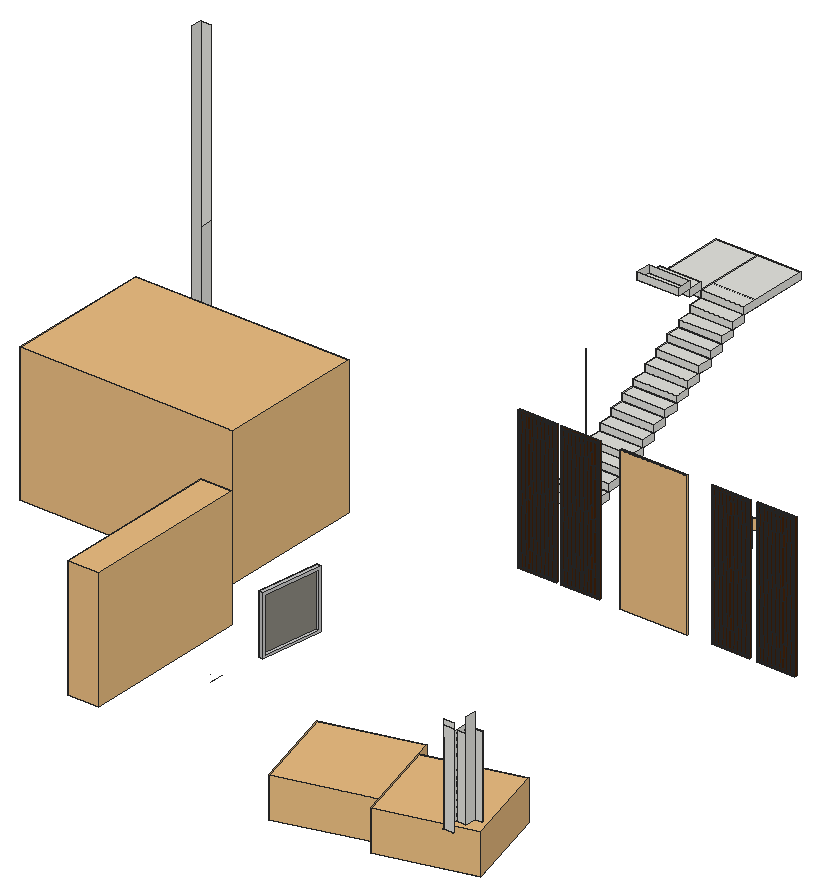
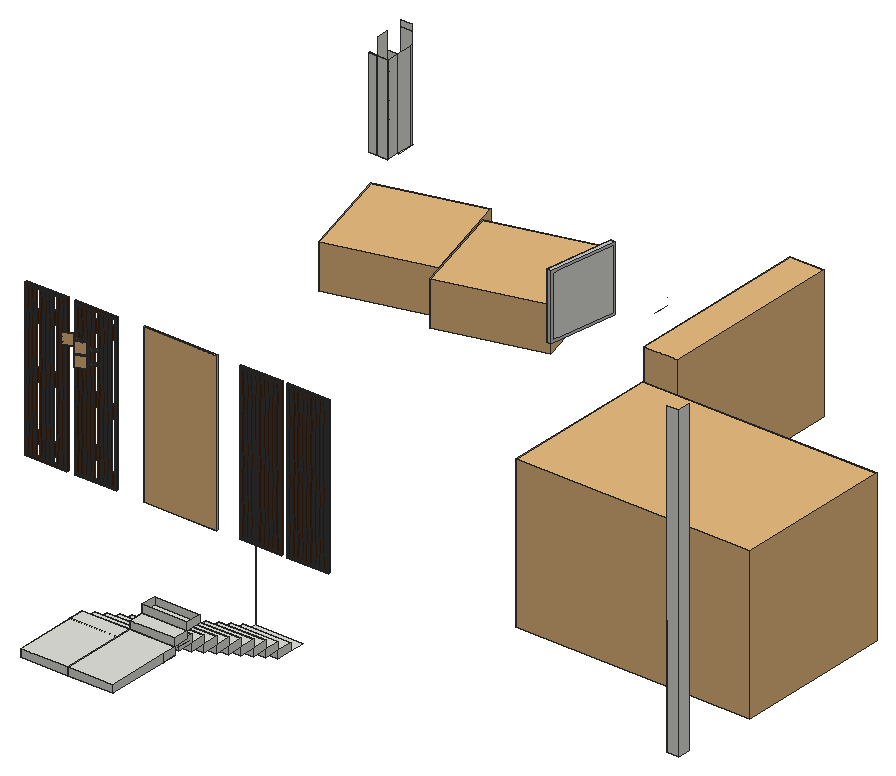
# SketchUp Ruby script. Lengths in inches.
U = 1.inch
M = Sketchup.active_model
def pt(a) = Geom::Point3d.new(a.map { |v| v * U })
def face(e, loops, mat)
  f = e.add_face(loops[0].map { |a| pt(a) })
  loops[1..].each { |l| e.add_face(l.map { |a| pt(a) }).erase! }
  f.material = f.back_material = mat if mat
  f
end
# faces: each face lists its corners as indices into pts; further lists are holes
def faces(e, pts, list, mat = nil) = list.each { |f| face(e, (f[0].is_a?(Array) ? f : [f]).map { |l| l.map { |i| pts[i] } }, mat) }
# xy, xz, yz: faces in a plane at the given z, y or x. An outline is a flat list of corners, or four numbers for a rectangle; further outlines are holes
def ring(l) = l.size == 4 ? [[l[0], l[1]], [l[2], l[1]], [l[2], l[3]], [l[0], l[3]]] : l.each_slice(2).to_a
def flat(e, list, mat, &to3) = list.each { |f| face(e, (f[0].is_a?(Array) ? f : [f]).map { |l| ring(l).map { |u, v| to3.(u, v) } }, mat) }
def xy(e, z, list, mat = nil) = flat(e, list, mat) { |x, y| [x, y, z] }
def xz(e, y, list, mat = nil) = flat(e, list, mat) { |x, z| [x, y, z] }
def yz(e, x, list, mat = nil) = flat(e, list, mat) { |y, z| [x, y, z] }
def lines(e, pts, list) = list.each { |a, b| e.add_line(pt(pts[a]), pt(pts[b])) }
# prism: a flat outline (further loops are holes) pulled along v
def prism(e, loops, v, mat = nil)
  f = face(e, loops, mat); d = Geom::Vector3d.new(v.map { |x| x * U })
  f.pushpull(f.normal.samedirection?(d) ? d.length : -d.length)
end
def box(e, o, s, mat = nil) = prism(e, [[o, [o[0] + s[0], o[1], o[2]], [o[0] + s[0], o[1] + s[1], o[2]], [o[0], o[1] + s[1], o[2]]]], [0, 0, s[2]], mat)
def at(x, y, z, deg = 0) = Geom::Transformation.translation(pt([x, y, z])) * Geom::Transformation.rotation(ORIGIN, Z_AXIS, deg.degrees)
def axes(o, x, y, z) = Geom::Transformation.new([*x, 0, *y, 0, *z, 0, *pt(o).to_a, 1])
def part(name) = M.definitions.add(name)
# library, detail: a bought-in or finely detailed component or shape, given as its bounding box
def library(name, o, s) = part(name).tap { |d| box(d.entities, o, s) }
def detail(e, o, s) = box(e.add_group.entities, o, s)
def put(e, d, t, mat = nil) = e.add_instance(d, t).tap { |i| i.material = mat if mat }
def group(e, t, mat = nil) = e.add_group.tap { |g| g.transformation = t; g.material = mat if mat }.entities
root = M.entities
M.materials.add("1797872045_ed86075bf6").color = [137, 134, 125]
M.materials.add("Copper_Blurry").color = [70, 35, 10]
M.materials.add("Mat3d66-543176-6-815").color = [163, 122, 73]
M.materials.add("[_0137_Black_]").color = [200, 200, 200]
c1 = library("VachCNC-038",[0,-0.94,0],[44.09,0.94,94.49])
c2 = part("Component\#7")
box(c2.entities,[0,0,-1],[2.125,8.03,1],"Copper_Blurry")
c3 = part("Component\#11")
box(c3.entities,[0,0,-1],[2,8.03,1],"Copper_Blurry")
c4 = part("Component\#9")
box(c4.entities,[0,0,-1],[2,8.03,1],"Copper_Blurry")
c5 = part("Component\#8")
box(c5.entities,[0,0,-0.75],[0.125,2,0.5],"Copper_Blurry")
c6 = part("Group\#54")
prism(c6.entities,[[[0,0,0],[0,96,0],[26,96,0],[26,0,0]],[[25.3125,0.6875,0],[25.3125,95.3125,0],[0.6875,95.3125,0],[0.6875,0.6875,0]]],[0,0,1],"Copper_Blurry")
prism(c6.entities,[[[0.8125,0.8125,0],[0.8125,95.1875,0],[25.1875,95.1875,0],[25.1875,0.8125,0]],[[24.5,1.5,0],[24.5,94.5,0],[1.5,94.5,0],[1.5,1.5,0]]],[0,0,1],"Copper_Blurry")
c7 = part("Component\#3")
box(c7.entities,[1,0,0],[0.5,93,1],"Copper_Blurry")
c8 = part("Group\#52")
put(c8.entities,c7,at(0.25,0,-1))
c9 = part("Group\#10")
put(c9.entities,c7,at(0.25,0,-1))
c10 = part("Group\#83")
put(c10.entities,c2,axes([16.75,83.45,1],[-1,0,0],[0,1,0],[0,0,1]))
put(c10.entities,c2,axes([22,79.4375,1],[-1,0,0],[0,1,0],[0,0,1]))
put(c10.entities,c2,axes([6.25,86.47,1],[-1,0,0],[0,1,0],[0,0,1]))
put(c10.entities,c2,at(14.625,50.02,1))
put(c10.entities,c2,at(19.875,47,1))
put(c10.entities,c2,at(17.25,42.98,1))
put(c10.entities,c2,at(4.125,34.97,1))
put(c10.entities,c2,at(9.375,48.02,1))
put(c10.entities,c2,at(1.5,38.98,1))
put(c10.entities,c2,at(12,41.98,1))
put(c10.entities,c2,at(6.75,44,1))
put(c10.entities,c2,axes([14.125,82.45,1],[-1,0,0],[0,1,0],[0,0,1]))
put(c10.entities,c3,at(22.5,39.97,1))
put(c10.entities,c2,axes([11.5,74.42,1],[-1,0,0],[0,1,0],[0,0,1]))
put(c10.entities,c2,at(1.5,1.5,1))
put(c10.entities,c2,at(19.875,16.5625,1))
put(c10.entities,c2,at(9.375,13.55,1))
put(c10.entities,c2,at(4.125,9.53,1))
put(c10.entities,c2,at(12,12.55,1))
put(c10.entities,c2,at(6.75,5.52,1))
put(c10.entities,c4,at(22.5,12.55,1))
put(c10.entities,c2,at(17.25,8.53,1))
put(c10.entities,c2,at(14.625,4.52,1))
put(c10.entities,c2,axes([3.625,82.45,1],[-1,0,0],[0,1,0],[0,0,1]))
put(c10.entities,c2,axes([19.375,75.42,1],[-1,0,0],[0,1,0],[0,0,1]))
put(c10.entities,c2,axes([8.875,78.4375,1],[-1,0,0],[0,1,0],[0,0,1]))
put(c10.entities,c4,axes([24.5,72.11,1],[-1,0,0],[0,1,0],[0,0,1]))
put(c10.entities,c5,at(25.1875,89.18,1))
put(c10.entities,c5,at(25.1875,4.6875,1))
put(c10.entities,c6,at(0,0,0))
put(c10.entities,c8,at(2.375,1.5,1))
put(c10.entities,c9,at(12.875,1.5,1))
put(c10.entities,c9,at(10.25,1.5,1))
put(c10.entities,c9,at(7.625,1.5,1))
put(c10.entities,c9,at(18.125,1.5,1))
put(c10.entities,c9,at(20.75,1.5,1))
put(c10.entities,c9,at(15.5,1.5,1))
put(c10.entities,c9,at(5,1.5,1))
c11 = library("Group\#144",[-12.96,-14.03,0],[79.67,79.67,34.25])
c12 = library("3D+ร้าน",[-61.68,-2.51,0],[183.73,124.56,118.11])
c13 = library("Wall+clothing+display+con+playwood+y+baldosas",[326.98,223.67,0],[26.48,142.21,102.3])
c14 = library("Group19",[-170.36,-43.1,0],[221.84,210,22])
c15 = library("Group14",[-165.46,-43.1,0],[221.84,210,22])
c16 = library("Group21",[-163.02,-39.7,0],[221.84,209.99,22])
xy(root,6,[[345.665,506.656,382.559,518.696],[382.559,518.696,382.5625,530.736]])
xy(root,12,[[345.665,518.696,382.559,530.736],[382.559,530.736,382.5625,542.776]])
xy(root,18,[[345.665,530.736,382.559,542.776],[382.559,542.776,382.5625,554.816]])
xy(root,24,[[345.665,542.776,382.559,554.816],[382.559,554.816,382.5625,566.856]])
xy(root,27.6875,[[55.762,494.368,64.762,494.743]])
xy(root,30,[[345.665,554.816,382.559,566.856],[382.559,566.856,382.5625,578.896]])
xy(root,36,[[345.665,566.856,382.559,578.896],[382.559,578.896,382.5625,590.936]])
xy(root,42,[[345.665,578.896,382.559,590.936],[382.559,590.936,382.5625,602.976]])
xy(root,48,[[345.665,590.936,382.559,602.976],[382.559,602.976,382.5625,615.016]])
xy(root,52.9375,[[627.244,47.656,628.181,47.692,636.315,48,628.181,48,628.181,61.6875,627.244,61.6875],[628.181,61.6875,636.315,70.552],[628.181,70.552,636.315,71.3125],[636.315,70.552,642.494,71.3125]])
xy(root,54,[[345.665,602.976,382.559,615.016],[382.559,615.016,382.5625,627.056]])
xy(root,60,[[345.665,615.016,382.559,627.056],[382.559,627.056,382.5625,639.096]])
xy(root,66,[[345.665,627.056,382.559,639.096],[382.559,639.096,382.5625,651.136]])
xy(root,72,[[345.665,639.096,382.559,651.136],[382.559,651.136,382.5625,663.176]])
xy(root,78,[[345.665,651.136,382.559,663.176],[382.559,663.176,382.5625,675.216]])
xy(root,84,[[345.665,663.176,345.668,675.216],[345.668,663.176,382.559,675.216],[310.55,675.216,310.612,687.256],[310.612,675.216,345.665,735.256],[382.559,675.216,382.5625,687.256],
  [310.55,687.256,310.612,735.256],[345.665,687.256,382.559,735.443]])
xy(root,90,[[310.55,663.216,310.612,675.216,345.665,675.216,345.665,663.216],[310.55,675.216,310.612,687.153],[310.612,675.216,345.665,675.216,345.665,735.256,310.55,735.256,310.55,687.153,310.612,687.153],[345.665,675.216,382.559,735.443]])
xy(root,96,[[310.55,651.216,310.612,663.216,345.665,663.216,345.665,651.216],[310.55,663.216,345.665,663.216,345.665,675.216,310.612,675.216]])
xz(root,48,[[628.181,52.9375,636.315,132],[628.181,52.9375,636.315,137]])
xz(root,61.6875,[[628.181,52.9375,636.315,122.249]])
xz(root,70.552,[[636.315,52.9375,642.431,122.249]])
xz(root,71.3125,[[628.181,52.9375,636.315,122.249],[628.181,52.9375,642.494,52.9375,642.493,122.249,628.181,122.249]])
xz(root,504,[[55.762,27.6875,64.762,269.1875]])
xz(root,506.656,[[382.549,6,382.559,132]])
xz(root,518.696,[[345.665,6,382.549,12],[382.549,6,382.559,12]])
xz(root,530.736,[[345.665,6,382.559,12],[345.665,12,382.549,18],[382.549,12,382.559,18]])
xz(root,542.776,[[345.665,12,382.559,18],[345.665,18,382.549,24],[382.549,18,382.559,24]])
xz(root,554.816,[[345.665,18,382.559,24],[345.665,24,382.549,30],[382.549,24,382.559,30]])
xz(root,566.856,[[345.665,24,382.559,30],[345.665,30,382.549,36],[382.549,30,382.559,36]])
xz(root,578.896,[[345.665,30,382.559,36],[345.665,36,382.549,42],[382.549,36,382.559,42]])
xz(root,590.936,[[345.665,36,382.559,42],[345.665,42,382.549,48],[382.549,42,382.559,48]])
xz(root,602.976,[[345.665,42,382.559,48],[345.665,48,382.549,54],[382.549,48,382.559,54]])
xz(root,615.016,[[345.665,48,382.559,54],[345.665,54,382.549,60],[382.549,54,382.559,60]])
xz(root,627.056,[[345.665,54,382.559,60],[345.665,60,382.549,66],[382.549,60,382.559,66]])
xz(root,639.096,[[345.665,60,382.559,66],[345.665,66,382.549,72],[382.549,66,382.559,72]])
xz(root,651.136,[[345.665,66,382.559,72],[345.665,72,382.549,78],[382.549,72,382.559,78]])
xz(root,651.216,[[310.55,96,345.665,102]])
xz(root,663.176,[[345.665,72,382.559,78],[345.665,78,382.549,84],[382.549,78,382.559,84]])
xz(root,663.216,[[310.55,90,345.665,96],[310.612,96,345.665,102]])
xz(root,675.216,[[345.665,78,382.559,84],[310.55,84,310.612,90],[310.612,84,345.665,90],[345.665,84,382.549,90],[382.549,84,382.559,90],
  [310.612,90,345.665,96]])
xz(root,687.256,[[345.665,84,382.559,90]])
xz(root,735.256,[[310.55,84,345.665,90]])
xz(root,735.443,[[345.665,84,382.559,90]])
yz(root,55.762,[[494.368,27.6875,504,269.1875]])
yz(root,64.762,[[494.125,27.6875,504,119.239]])
yz(root,310.55,[[687.256,84,735.256,90]])
yz(root,310.612,[[675.216,84,687.256,84,687.153,90,675.216,90]])
yz(root,345.665,[[518.696,6,530.736,12],[530.736,12,542.776,18],[542.776,18,554.816,24],[554.816,24,566.856,30],[566.856,30,578.896,36],
  [578.896,36,590.936,42],[590.936,42,602.976,48],[602.976,48,615.016,54],[615.016,54,627.056,60],[627.056,60,639.096,66],
  [639.096,66,651.136,72],[651.136,72,663.176,78],[663.176,78,675.216,84],[675.216,84,687.256,90],[687.256,84,735.256,90],
  [735.256,84,735.443,90],[663.216,90,675.216,96],[651.216,96,663.216,102]])
yz(root,382.559,[[518.696,6,530.736,12],[530.736,12,542.776,18],[542.776,18,554.816,24],[554.816,24,566.856,30],[566.856,30,578.896,36],
  [578.896,36,590.936,42],[590.936,42,602.976,48],[602.976,48,615.016,54],[615.016,54,627.056,60],[627.056,60,639.096,66],
  [639.096,66,651.136,72],[651.136,72,663.176,78],[663.176,78,675.216,84],[675.216,84,735.443,90]])
yz(root,628.181,[[48,52.9375,49.975,122.249],[49.975,52.9375,61.6875,122.249],[61.6875,52.9375,70.552,122.249],[70.552,52.9375,71.3125,122.249]])
yz(root,636.315,[[61.6875,52.9375,61.6875,135.296,70.553,135.296,70.552,132.875,70.552,52.9375],[61.6875,52.9375,70.552,122.249],[70.552,52.9375,71.3125,122.249]])
p = [[310.55,687.256,84],[310.55,687.153,90],[310.612,687.153,90],[310.612,687.256,84],[310.612,675.216,90],[310.55,663.216,90],
  [310.55,663.216,96],[310.612,675.216,96],[310.612,663.216,96],[310.55,651.216,96],[310.55,651.216,102],[310.612,663.216,102],
  [382.549,554.816,24],[382.549,557.816,24],[382.549,566.856,30],[382.549,569.856,30],[382.549,578.896,36],[382.549,581.896,36],
  [382.549,590.936,42],[382.549,593.936,42],[382.549,602.976,48],[382.549,605.976,48],[382.549,615.016,54],[382.549,618.016,54],
  [382.549,627.056,60],[382.549,630.056,60],[382.549,639.096,66],[382.549,642.096,66],[382.549,651.136,72],[382.549,654.136,72],
  [382.549,663.176,78],[382.549,666.176,78],[382.549,675.216,84],[382.549,678.216,84],[308.77,663.176,90],[308.77,675.216,90],
  [345.665,663.176,84],[345.655,663.176,84],[382.471,106.619,52.909],[382.458,106.619,52.909],[382.468,118.659,52.909],[382.471,118.659,52.909],
  [382.468,106.619,58.909],[382.458,106.619,58.909],[345.665,663.176,90],[345.655,663.176,90],[345.655,666.176,84],[310.55,675.302,96],
  [310.612,675.302,96],[310.55,675.404,96],[382.549,542.776,18],[382.549,545.776,18],[382.549,530.736,12],[382.549,533.736,12],
  [382.549,518.696,6],[382.549,521.696,6]]
faces(root,p,[[0,1,2,3],[4,5,6,7],[8,9,10,11]])
lines(root,p,[[12,13],[14,15],[16,17],[18,19],[20,21],[22,23],[24,25],[26,27],[28,29],[30,31],[32,33],[34,35],
  [36,37],[38,39],[40,41],[42,43],[44,45],[37,46],[41,38],[47,48],[47,49],[50,51],[52,53],[54,55]])
put(root,c1,axes([477.6,425.38,2.61],[1.29,0,0],[0,1.29,0],[0,0,1.29]))
put(root,c10,axes([426.61,425.93,3.17],[1.26126,0,0],[0,0,1.26126],[0,-1.26126,0]))
put(root,c10,axes([390.25,425.93,3.17],[1.26126,0,0],[0,0,1.26126],[0,-1.26126,0]))
g1 = group(root,at(593.62,425.93,3.17))
put(g1,c2,axes([21.125,-1.26,105.26],[-1.26126,0,0],[0,0,1.26126],[0,-1.26126,0]))
put(g1,c2,axes([27.75,-1.26,100.19],[-1.26126,0,0],[0,0,1.26126],[0,-1.26126,0]))
put(g1,c2,axes([7.88,-1.26,109.06],[-1.26126,0,0],[0,0,1.26126],[0,-1.26126,0]))
put(g1,c2,axes([18.45,-1.26,63.08],[1.26126,0,0],[0,0,1.26126],[0,-1.26126,0]))
put(g1,c2,axes([25.07,-1.26,59.28],[1.26126,0,0],[0,0,1.26126],[0,-1.26126,0]))
put(g1,c2,axes([21.76,-1.26,54.21],[1.26126,0,0],[0,0,1.26126],[0,-1.26126,0]))
put(g1,c2,axes([5.2,-1.26,44.11],[1.26126,0,0],[0,0,1.26126],[0,-1.26126,0]))
put(g1,c2,axes([11.82,-1.26,60.56],[1.26126,0,0],[0,0,1.26126],[0,-1.26126,0]))
put(g1,c2,axes([1.89,-1.26,49.17],[1.26126,0,0],[0,0,1.26126],[0,-1.26126,0]))
put(g1,c2,axes([15.14,-1.26,52.95],[1.26126,0,0],[0,0,1.26126],[0,-1.26126,0]))
put(g1,c2,axes([8.51,-1.26,55.5],[1.26126,0,0],[0,0,1.26126],[0,-1.26126,0]))
put(g1,c2,axes([17.82,-1.26,104],[-1.26126,0,0],[0,0,1.26126],[0,-1.26126,0]))
put(g1,c3,axes([28.38,-1.26,50.41],[1.26126,0,0],[0,0,1.26126],[0,-1.26126,0]))
put(g1,c2,axes([14.5,-1.26,93.87],[-1.26126,0,0],[0,0,1.26126],[0,-1.26126,0]))
put(g1,c2,axes([1.89,-1.26,1.89],[1.26126,0,0],[0,0,1.26126],[0,-1.26126,0]))
put(g1,c2,axes([25.07,-1.26,20.89],[1.26126,0,0],[0,0,1.26126],[0,-1.26126,0]))
put(g1,c2,axes([11.82,-1.26,17.09],[1.26126,0,0],[0,0,1.26126],[0,-1.26126,0]))
put(g1,c2,axes([5.2,-1.26,12.02],[1.26126,0,0],[0,0,1.26126],[0,-1.26126,0]))
put(g1,c2,axes([15.14,-1.26,15.82],[1.26126,0,0],[0,0,1.26126],[0,-1.26126,0]))
put(g1,c2,axes([8.51,-1.26,6.96],[1.26126,0,0],[0,0,1.26126],[0,-1.26126,0]))
put(g1,c4,axes([28.38,-1.26,15.82],[1.26126,0,0],[0,0,1.26126],[0,-1.26126,0]))
put(g1,c2,axes([21.76,-1.26,10.76],[1.26126,0,0],[0,0,1.26126],[0,-1.26126,0]))
put(g1,c2,axes([18.45,-1.26,5.7],[1.26126,0,0],[0,0,1.26126],[0,-1.26126,0]))
put(g1,c2,axes([4.57,-1.26,104],[-1.26126,0,0],[0,0,1.26126],[0,-1.26126,0]))
put(g1,c2,axes([24.4375,-1.26,95.13],[-1.26126,0,0],[0,0,1.26126],[0,-1.26126,0]))
put(g1,c2,axes([11.19,-1.26,98.93],[-1.26126,0,0],[0,0,1.26126],[0,-1.26126,0]))
put(g1,c4,axes([30.9,-1.26,90.94],[-1.26126,0,0],[0,0,1.26126],[0,-1.26126,0]))
put(g1,c5,axes([31.77,-1.26,112.48],[1.26126,0,0],[0,0,1.26126],[0,-1.26126,0]))
put(g1,c5,axes([31.77,-1.26,5.91],[1.26126,0,0],[0,0,1.26126],[0,-1.26126,0]))
put(g1,c6,axes([0,0,0],[1.26126,0,0],[0,0,1.26126],[0,-1.26126,0]))
put(g1,c8,axes([3,-1.26,1.89],[1.26126,0,0],[0,0,1.26126],[0,-1.26126,0]))
put(g1,c9,axes([16.24,-1.26,1.89],[1.26126,0,0],[0,0,1.26126],[0,-1.26126,0]))
put(g1,c9,axes([12.93,-1.26,1.89],[1.26126,0,0],[0,0,1.26126],[0,-1.26126,0]))
put(g1,c9,axes([9.62,-1.26,1.89],[1.26126,0,0],[0,0,1.26126],[0,-1.26126,0]))
put(g1,c9,axes([22.86,-1.26,1.89],[1.26126,0,0],[0,0,1.26126],[0,-1.26126,0]))
put(g1,c9,axes([26.17,-1.26,1.89],[1.26126,0,0],[0,0,1.26126],[0,-1.26126,0]))
put(g1,c9,axes([19.55,-1.26,1.89],[1.26126,0,0],[0,0,1.26126],[0,-1.26126,0]))
put(g1,c9,axes([6.31,-1.26,1.89],[1.26126,0,0],[0,0,1.26126],[0,-1.26126,0]))
g2 = group(root,at(555.04,425.93,3.17))
put(g2,c2,axes([21.125,-1.26,105.26],[-1.26126,0,0],[0,0,1.26126],[0,-1.26126,0]))
put(g2,c2,axes([27.75,-1.26,100.19],[-1.26126,0,0],[0,0,1.26126],[0,-1.26126,0]))
put(g2,c2,axes([7.88,-1.26,109.06],[-1.26126,0,0],[0,0,1.26126],[0,-1.26126,0]))
put(g2,c2,axes([18.45,-1.26,63.08],[1.26126,0,0],[0,0,1.26126],[0,-1.26126,0]))
put(g2,c2,axes([25.07,-1.26,59.28],[1.26126,0,0],[0,0,1.26126],[0,-1.26126,0]))
put(g2,c2,axes([21.76,-1.26,54.21],[1.26126,0,0],[0,0,1.26126],[0,-1.26126,0]))
put(g2,c2,axes([5.2,-1.26,44.11],[1.26126,0,0],[0,0,1.26126],[0,-1.26126,0]))
put(g2,c2,axes([11.82,-1.26,60.56],[1.26126,0,0],[0,0,1.26126],[0,-1.26126,0]))
put(g2,c2,axes([1.89,-1.26,49.17],[1.26126,0,0],[0,0,1.26126],[0,-1.26126,0]))
put(g2,c2,axes([15.14,-1.26,52.95],[1.26126,0,0],[0,0,1.26126],[0,-1.26126,0]))
put(g2,c2,axes([8.51,-1.26,55.5],[1.26126,0,0],[0,0,1.26126],[0,-1.26126,0]))
put(g2,c2,axes([17.82,-1.26,104],[-1.26126,0,0],[0,0,1.26126],[0,-1.26126,0]))
put(g2,c3,axes([28.38,-1.26,50.41],[1.26126,0,0],[0,0,1.26126],[0,-1.26126,0]))
put(g2,c2,axes([14.5,-1.26,93.87],[-1.26126,0,0],[0,0,1.26126],[0,-1.26126,0]))
put(g2,c2,axes([1.89,-1.26,1.89],[1.26126,0,0],[0,0,1.26126],[0,-1.26126,0]))
put(g2,c2,axes([25.07,-1.26,20.89],[1.26126,0,0],[0,0,1.26126],[0,-1.26126,0]))
put(g2,c2,axes([11.82,-1.26,17.09],[1.26126,0,0],[0,0,1.26126],[0,-1.26126,0]))
put(g2,c2,axes([5.2,-1.26,12.02],[1.26126,0,0],[0,0,1.26126],[0,-1.26126,0]))
put(g2,c2,axes([15.14,-1.26,15.82],[1.26126,0,0],[0,0,1.26126],[0,-1.26126,0]))
put(g2,c2,axes([8.51,-1.26,6.96],[1.26126,0,0],[0,0,1.26126],[0,-1.26126,0]))
put(g2,c4,axes([28.38,-1.26,15.82],[1.26126,0,0],[0,0,1.26126],[0,-1.26126,0]))
put(g2,c2,axes([21.76,-1.26,10.76],[1.26126,0,0],[0,0,1.26126],[0,-1.26126,0]))
put(g2,c2,axes([18.45,-1.26,5.7],[1.26126,0,0],[0,0,1.26126],[0,-1.26126,0]))
put(g2,c2,axes([4.57,-1.26,104],[-1.26126,0,0],[0,0,1.26126],[0,-1.26126,0]))
put(g2,c2,axes([24.4375,-1.26,95.13],[-1.26126,0,0],[0,0,1.26126],[0,-1.26126,0]))
put(g2,c2,axes([11.19,-1.26,98.93],[-1.26126,0,0],[0,0,1.26126],[0,-1.26126,0]))
put(g2,c4,axes([30.9,-1.26,90.94],[-1.26126,0,0],[0,0,1.26126],[0,-1.26126,0]))
put(g2,c5,axes([31.77,-1.26,112.48],[1.26126,0,0],[0,0,1.26126],[0,-1.26126,0]))
put(g2,c5,axes([31.77,-1.26,5.91],[1.26126,0,0],[0,0,1.26126],[0,-1.26126,0]))
put(g2,c6,axes([0,0,0],[1.26126,0,0],[0,0,1.26126],[0,-1.26126,0]))
put(g2,c8,axes([3,-1.26,1.89],[1.26126,0,0],[0,0,1.26126],[0,-1.26126,0]))
put(g2,c9,axes([16.24,-1.26,1.89],[1.26126,0,0],[0,0,1.26126],[0,-1.26126,0]))
put(g2,c9,axes([12.93,-1.26,1.89],[1.26126,0,0],[0,0,1.26126],[0,-1.26126,0]))
put(g2,c9,axes([9.62,-1.26,1.89],[1.26126,0,0],[0,0,1.26126],[0,-1.26126,0]))
put(g2,c9,axes([22.86,-1.26,1.89],[1.26126,0,0],[0,0,1.26126],[0,-1.26126,0]))
put(g2,c9,axes([26.17,-1.26,1.89],[1.26126,0,0],[0,0,1.26126],[0,-1.26126,0]))
put(g2,c9,axes([19.55,-1.26,1.89],[1.26126,0,0],[0,0,1.26126],[0,-1.26126,0]))
put(g2,c9,axes([6.31,-1.26,1.89],[1.26126,0,0],[0,0,1.26126],[0,-1.26126,0]))
put(root,c11,at(535.43,82.36,4,105))
put(root,c11,at(616.71,89.38,4.17,105))
put(root,c12,axes([137.26,288.51,5.43],[0.99,0,0],[0,0.99,0],[0,0,0.99]))
put(root,c13,at(-56.875,-129.32,9.34))
g3 = group(root,at(397.05,143.52,59.4))
xy(g3,0,[[0,0,-3.95,0.57,3.66,53.38,7.61,52.81]],"[_0137_Black_]")
xy(g3,2,[[-2.875,2.43,-3.67,2.55,3.375,51.4,4.17,51.29]],"1797872045_ed86075bf6")
xy(g3,2,[[0.28,1.98,7.33,50.83,3.375,51.4,-3.67,2.55]],"[_0137_Black_]")
xy(g3,48.6,[[-2.875,2.43,4.17,51.29,3.375,51.4,-3.67,2.55]],"1797872045_ed86075bf6")
xy(g3,48.6,[[0.28,1.98,-3.67,2.55,3.375,51.4,7.33,50.83]],"[_0137_Black_]")
xy(g3,50.59,[[0,0,7.61,52.81,3.66,53.38,-3.95,0.57]],"[_0137_Black_]")
p = [[-3.95,0.57,50.59],[-3.95,0.57,0],[0,0,0],[0,0,50.59],[7.61,52.81,50.59],[7.61,52.81,0],
  [7.33,50.83,2],[0.28,1.98,2],[0.28,1.98,48.6],[7.33,50.83,48.6],[3.66,53.38,50.59],[3.66,53.38,0],
  [-3.67,2.55,2],[3.375,51.4,2],[3.375,51.4,48.6],[-3.67,2.55,48.6],[-2.875,2.43,2],[-2.875,2.43,48.6],
  [4.17,51.29,2],[4.17,51.29,48.6]]
faces(g3,p,[[0,1,2,3],[[4,3,2,5],[6,7,8,9]],[[0,10,11,1],[12,13,14,15]],[11,10,4,5],[12,15,8,7],[14,13,6,9]],"[_0137_Black_]")
faces(g3,p,[[15,12,16,17],[16,18,19,17],[13,14,19,18]],"1797872045_ed86075bf6")
faces(g3,p,[[13,12,15,14]])
put(root,c14,axes([581.64,432.34,84.76],[0,0,-0.03937],[-0.037,-0.01347,0],[0.01347,-0.037,0]))
g4 = group(root,at(573.91,429.28,79.83))
p = [[1.12,0.41,4.32],[2.61,0.95,3.125],[1.17,0.43,10.33],[1.47,0.54,3.66],[4.17,1.52,3.25],[1.63,0.59,3.12],
  [1.55,0.36,3.62],[1.7,0.41,3.12],[3.78,1.16,3.21],[1.18,0.22,10.25],[5.84,1.91,3.59],[1.24,0.24,4.24],
  [5.61,2.04,3.53],[6.54,2.38,3.89],[7.22,2.42,4.22],[3.71,1.35,11.32],[5.77,2.1,10.9375],[7.16,2.6,10.31],
  [7.39,2.6875,4.35],[0.62,0.02,9.61],[0.68,0.04,4.91],[2.68,0.77,11.4],[4.24,1.33,11.28],[5.68,1.86,11],
  [6.61,2.2,10.64],[7.45,2.5,10.18],[8.16,2.76,9.62],[8.21,2.78,4.96],[8.09,2.95,4.91],[0.55,0.2,4.96],
  [0.61,0.22,9.66],[8.15,2.96,9.57],[-0.35,-0.34,5.68],[8.71,3.17,5.66],[-0.18,-0.07,5.54],[8.85,3.01,5.8],
  [-1.06,-0.38,6.03],[-0.42,-0.15,8.89],[-0.99,-0.57,8.54],[-1.79,-0.86,6.33],[-0.11,-0.25,9.03],[8.78,3.2,8.73],
  [9.0625,3.3,6.45],[8.78,2.99,8.87],[9.13,3.11,8.08],[9.18,3.13,6.65],[-2.02,-0.74,6.39],[-1.86,-0.68,8.24],
  [-3.41,-1.45,6.68],[-3.49,-1.27,6.68],[-3.42,-1.45,7.89],[-1.95,-0.92,8.18],[9.1875,3.34,7.26],[-6.06,-2.2,6.8125],
  [-5.98,-2.39,6.8125],[-3.48,-1.27,7.89],[9.25,3.16,7.27],[-5.99,-2.39,7.76],[-6.05,-2.2,7.76],[9.11,3.32,7.88],
  [1.54,0.35,10.91],[1.49,0.54,10.95],[1.7,0.41,11.41],[1.63,0.59,11.41]]
faces(g4,p,[[0,1,2],[0,3,1],[1,4,2],[5,3,6],[1,5,7],[6,7,5],[8,7,6],[7,8,1],
  [3,5,1],[4,1,8],[9,10,8],[9,8,11],[8,6,11],[8,10,4],[4,12,2],[12,4,10],
  [12,13,2],[13,12,10],[9,14,10],[11,6,3],[10,14,13],[3,0,11],[13,15,2],[13,16,15],
  [13,17,16],[18,13,14],[13,18,17],[19,11,20],[19,9,11],[20,11,0],[9,21,14],[21,22,14],
  [22,23,14],[23,24,14],[24,25,14],[26,27,14],[25,26,14],[28,18,14],[14,27,28],[0,29,20],
  [0,2,30],[29,0,30],[18,31,17],[18,28,31],[19,20,32],[32,20,29],[33,28,27],[28,33,31],
  [29,34,32],[34,29,30],[26,35,27],[27,35,33],[34,36,32],[36,34,37],[34,30,37],[38,32,39],
  [39,32,36],[38,40,32],[40,19,32],[33,41,31],[42,33,35],[33,42,41],[26,43,35],[43,44,35],
  [44,45,35],[35,45,42],[36,46,39],[46,36,47],[36,37,47],[48,39,49],[50,39,48],[50,51,39],
  [46,49,39],[51,38,39],[49,46,47],[52,42,45],[42,52,41],[49,53,54],[50,48,54],[54,48,49],
  [53,49,55],[49,47,55],[44,56,45],[45,56,52],[57,54,53],[53,58,57],[57,50,54],[53,55,58],
  [56,44,59],[52,59,41],[59,52,56],[50,57,58],[58,55,50],[55,47,50],[51,50,47],[41,59,44],
  [44,43,41],[38,51,47],[47,37,38],[40,38,37],[31,41,43],[19,40,37],[37,30,19],[43,26,31],
  [9,19,30],[26,25,17],[17,31,26],[30,2,9],[25,24,17],[9,60,21],[60,9,2],[15,61,2],
  [2,61,60],[16,17,24],[24,23,16],[62,60,61],[60,62,21],[61,63,62],[15,63,61],[15,16,22],
  [23,22,16],[63,15,21],[22,21,15],[21,62,63]],"Mat3d66-543176-6-815")
put(root,c15,axes([581.64,432.34,94.65],[0,0,-0.03937],[-0.037,-0.01347,0],[0.01347,-0.037,0]))
g5 = group(root,at(573.91,429.28,89.72))
xy(g5,2.93,[[1.7,0.41,2.61,0.95,1.63,0.59]],"Mat3d66-543176-6-815")
p = [[1.12,0.41,4.125],[2.61,0.95,2.93],[1.17,0.43,10.14],[1.47,0.54,3.46],[4.17,1.52,3.0625],[1.63,0.59,2.93],
  [1.55,0.36,3.43],[1.7,0.41,2.93],[3.78,1.16,3.02],[1.18,0.22,10.06],[5.84,1.91,3.4],[1.24,0.24,4.04],
  [5.61,2.04,3.34],[6.54,2.38,3.69],[7.22,2.42,4.03],[3.71,1.35,11.125],[5.77,2.1,10.74],[7.16,2.6,10.12],
  [7.39,2.6875,4.16],[0.62,0.02,9.41],[0.68,0.04,4.72],[2.68,0.77,11.21],[4.24,1.33,11.08],[5.68,1.86,10.8],
  [6.61,2.2,10.45],[7.45,2.5,9.98],[8.16,2.76,9.43],[8.21,2.78,4.77],[8.09,2.95,4.72],[0.55,0.2,4.77],
  [0.61,0.22,9.47],[8.15,2.96,9.38],[-0.35,-0.34,5.49],[8.71,3.17,5.47],[-0.18,-0.07,5.35],[8.85,3.01,5.6],
  [-1.06,-0.38,5.83],[-0.42,-0.15,8.7],[-0.99,-0.57,8.35],[-1.79,-0.86,6.14],[-0.11,-0.25,8.83],[8.78,3.2,8.54],
  [9.0625,3.3,6.26],[8.78,2.99,8.68],[9.13,3.11,7.89],[9.18,3.13,6.46],[-2.02,-0.74,6.2],[-1.86,-0.68,8.05],
  [-3.41,-1.45,6.49],[-3.49,-1.27,6.48],[-3.42,-1.45,7.7],[-1.95,-0.92,7.99],[9.1875,3.34,7.0625],[-6.06,-2.2,6.62],
  [-5.98,-2.39,6.62],[-3.48,-1.27,7.7],[9.25,3.16,7.08],[-5.99,-2.39,7.5625],[-6.05,-2.2,7.5625],[9.11,3.32,7.68],
  [1.54,0.35,10.72],[1.49,0.54,10.75],[1.7,0.41,11.22],[1.63,0.59,11.22]]
faces(g5,p,[[0,1,2],[0,3,1],[1,4,2],[5,3,6],[6,7,5],[8,7,6],[7,8,1],[3,5,1],
  [4,1,8],[9,10,8],[9,8,11],[8,6,11],[8,10,4],[4,12,2],[12,4,10],[12,13,2],
  [13,12,10],[9,14,10],[11,6,3],[10,14,13],[3,0,11],[13,15,2],[13,16,15],[13,17,16],
  [18,13,14],[13,18,17],[19,11,20],[19,9,11],[20,11,0],[9,21,14],[21,22,14],[22,23,14],
  [23,24,14],[24,25,14],[26,27,14],[25,26,14],[28,18,14],[14,27,28],[0,29,20],[0,2,30],
  [29,0,30],[18,31,17],[18,28,31],[19,20,32],[32,20,29],[33,28,27],[28,33,31],[29,34,32],
  [34,29,30],[26,35,27],[27,35,33],[34,36,32],[36,34,37],[34,30,37],[38,32,39],[39,32,36],
  [38,40,32],[40,19,32],[33,41,31],[42,33,35],[33,42,41],[26,43,35],[43,44,35],[44,45,35],
  [35,45,42],[36,46,39],[46,36,47],[36,37,47],[48,39,49],[50,39,48],[50,51,39],[46,49,39],
  [51,38,39],[49,46,47],[52,42,45],[42,52,41],[49,53,54],[50,48,54],[54,48,49],[53,49,55],
  [49,47,55],[44,56,45],[45,56,52],[57,54,53],[53,58,57],[57,50,54],[53,55,58],[56,44,59],
  [52,59,41],[59,52,56],[50,57,58],[58,55,50],[55,47,50],[51,50,47],[41,59,44],[44,43,41],
  [38,51,47],[47,37,38],[40,38,37],[31,41,43],[19,40,37],[37,30,19],[43,26,31],[9,19,30],
  [26,25,17],[17,31,26],[30,2,9],[25,24,17],[9,60,21],[60,9,2],[15,61,2],[2,61,60],
  [16,17,24],[24,23,16],[62,60,61],[60,62,21],[15,16,22],[23,22,16],[61,63,62],[15,63,61],
  [63,15,21],[22,21,15],[21,62,63]],"Mat3d66-543176-6-815")
put(root,c16,axes([589.46,435.1875,99.57],[0,0,-0.03937],[-0.037,-0.01347,0],[0.01347,-0.037,0]))
g6 = group(root,at(581.73,432.12,94.65))
p = [[1.5,0.55,2.83],[1.35,0.49,3.37],[1.43,0.31,3.33],[1.57,0.36,2.83],[3.65,1.12,2.92],[0.99,0.36,4.03],
  [2.48,0.9,2.84],[1.05,0.38,10.04],[4.04,1.47,2.96],[1.06,0.18,9.96],[5.71,1.87,3.3],[1.11,0.2,3.95],
  [5.49,2,3.25],[6.42,2.34,3.6],[7.1,2.375,3.93],[3.58,1.3,11.03],[5.64,2.05,10.65],[7.03,2.56,10.02],
  [7.26,2.64,4.0625],[0.5,-0.03,9.32],[0.55,-0.01,4.62],[2.55,0.72,11.11],[4.11,1.29,10.99],[5.55,1.8125,10.71],
  [6.48,2.15,10.35],[7.33,2.46,9.89],[8.03,2.71,9.33],[8.09,2.73,4.67],[7.97,2.9,4.62],[0.43,0.16,4.68],
  [0.48,0.18,9.37],[8.02,2.92,9.28],[-0.48,-0.38,5.39],[8.58,3.125,5.37],[-0.31,-0.11,5.25],[8.72,2.97,5.51],
  [-1.18,-0.43,5.74],[-0.55,-0.2,8.6],[-1.11,-0.61,8.25],[-1.91,-0.91,6.04],[-0.24,-0.3,8.74],[8.66,3.15,8.44],
  [8.9375,3.25,6.16],[8.65,2.9375,8.58],[9,3.07,7.79],[9.05,3.09,6.36],[-2.15,-0.78,6.1],[-1.98,-0.72,7.95],
  [-3.53,-1.5,6.39],[-3.61,-1.32,6.39],[-3.55,-1.5,7.6],[-2.08,-0.97,7.89],[9.0625,3.3,6.97],[-6.18,-2.25,6.52],
  [-6.11,-2.43,6.52],[-3.6,-1.3125,7.6],[9.13,3.11,6.99],[-6.11,-2.43,7.47],[-6.18,-2.25,7.47],[8.99,3.27,7.59],
  [1.41,0.31,10.62],[1.36,0.5,10.66],[1.57,0.36,11.12],[1.51,0.55,11.12]]
faces(g6,p,[[0,1,2],[2,3,0],[4,3,2],[5,6,7],[5,1,6],[6,8,7],[6,0,3],[3,4,6],
  [1,0,6],[8,6,4],[9,10,4],[9,4,11],[4,2,11],[4,10,8],[8,12,7],[12,8,10],
  [12,13,7],[13,12,10],[9,14,10],[11,2,1],[10,14,13],[1,5,11],[13,15,7],[13,16,15],
  [13,17,16],[18,13,14],[13,18,17],[19,11,20],[19,9,11],[20,11,5],[9,21,14],[21,22,14],
  [22,23,14],[23,24,14],[24,25,14],[26,27,14],[25,26,14],[28,18,14],[14,27,28],[5,29,20],
  [29,5,30],[5,7,30],[18,31,17],[18,28,31],[19,20,32],[32,20,29],[33,28,27],[28,33,31],
  [29,34,32],[34,29,30],[26,35,27],[27,35,33],[34,36,32],[36,34,37],[34,30,37],[38,32,39],
  [39,32,36],[38,40,32],[40,19,32],[33,41,31],[42,33,35],[33,42,41],[26,43,35],[43,44,35],
  [44,45,35],[35,45,42],[36,46,39],[46,36,47],[36,37,47],[48,39,49],[50,39,48],[50,51,39],
  [46,49,39],[51,38,39],[49,46,47],[52,42,45],[42,52,41],[49,53,54],[50,48,54],[54,48,49],
  [53,49,55],[49,47,55],[44,56,45],[45,56,52],[57,54,53],[53,58,57],[57,50,54],[53,55,58],
  [56,44,59],[59,52,56],[52,59,41],[50,57,58],[58,55,50],[55,47,50],[51,50,47],[41,59,44],
  [44,43,41],[38,51,47],[47,37,38],[40,38,37],[31,41,43],[19,40,37],[37,30,19],[43,26,31],
  [9,19,30],[26,25,17],[17,31,26],[30,7,9],[25,24,17],[60,9,7],[9,60,21],[7,61,60],
  [15,61,7],[16,17,24],[24,23,16],[62,60,61],[60,62,21],[15,16,22],[23,22,16],[61,63,62],
  [15,63,61],[63,15,21],[22,21,15],[21,62,63]],"Mat3d66-543176-6-815")
